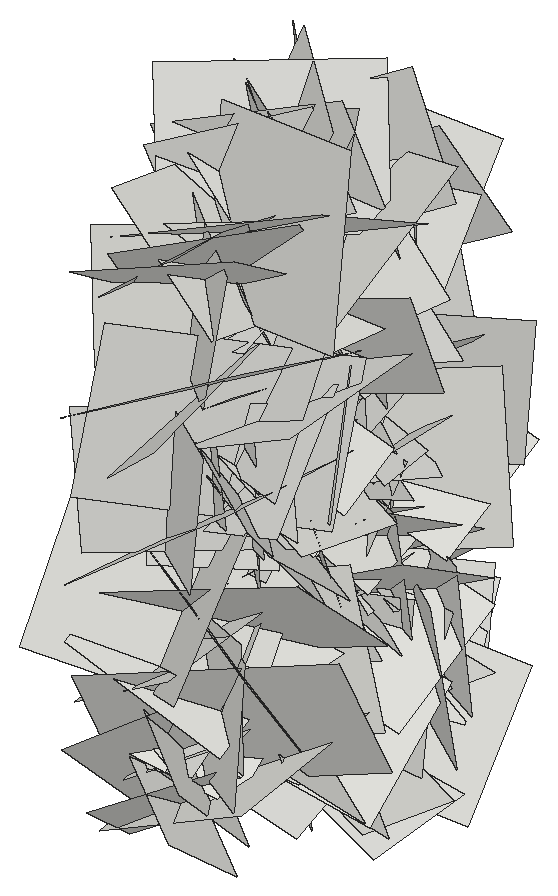
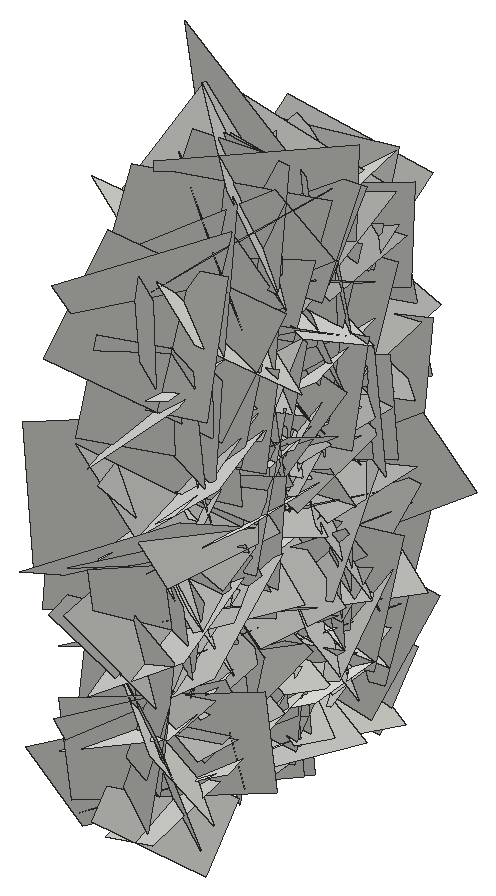
# SketchUp Ruby script. Lengths in inches.
U = 1.inch
M = Sketchup.active_model
def pt(a) = Geom::Point3d.new(a.map { |v| v * U })
def face(e, loops, mat)
  f = e.add_face(loops[0].map { |a| pt(a) })
  loops[1..].each { |l| e.add_face(l.map { |a| pt(a) }).erase! }
  f.material = f.back_material = mat if mat
  f
end
# faces: each face lists its corners as indices into pts; further lists are holes
def faces(e, pts, list, mat = nil) = list.each { |f| face(e, (f[0].is_a?(Array) ? f : [f]).map { |l| l.map { |i| pts[i] } }, mat) }
# xy, xz, yz: faces in a plane at the given z, y or x. An outline is a flat list of corners, or four numbers for a rectangle; further outlines are holes
def ring(l) = l.size == 4 ? [[l[0], l[1]], [l[2], l[1]], [l[2], l[3]], [l[0], l[3]]] : l.each_slice(2).to_a
def flat(e, list, mat, &to3) = list.each { |f| face(e, (f[0].is_a?(Array) ? f : [f]).map { |l| ring(l).map { |u, v| to3.(u, v) } }, mat) }
def xy(e, z, list, mat = nil) = flat(e, list, mat) { |x, y| [x, y, z] }
def xz(e, y, list, mat = nil) = flat(e, list, mat) { |x, z| [x, y, z] }
def yz(e, x, list, mat = nil) = flat(e, list, mat) { |y, z| [x, y, z] }
def lines(e, pts, list) = list.each { |a, b| e.add_line(pt(pts[a]), pt(pts[b])) }
# prism: a flat outline (further loops are holes) pulled along v
def prism(e, loops, v, mat = nil)
  f = face(e, loops, mat); d = Geom::Vector3d.new(v.map { |x| x * U })
  f.pushpull(f.normal.samedirection?(d) ? d.length : -d.length)
end
def box(e, o, s, mat = nil) = prism(e, [[o, [o[0] + s[0], o[1], o[2]], [o[0] + s[0], o[1] + s[1], o[2]], [o[0], o[1] + s[1], o[2]]]], [0, 0, s[2]], mat)
def at(x, y, z, deg = 0) = Geom::Transformation.translation(pt([x, y, z])) * Geom::Transformation.rotation(ORIGIN, Z_AXIS, deg.degrees)
def axes(o, x, y, z) = Geom::Transformation.new([*x, 0, *y, 0, *z, 0, *pt(o).to_a, 1])
def part(name) = M.definitions.add(name)
# library, detail: a bought-in or finely detailed component or shape, given as its bounding box
def library(name, o, s) = part(name).tap { |d| box(d.entities, o, s) }
def detail(e, o, s) = box(e.add_group.entities, o, s)
def put(e, d, t, mat = nil) = e.add_instance(d, t).tap { |i| i.material = mat if mat }
def group(e, t, mat = nil) = e.add_group.tap { |g| g.transformation = t; g.material = mat if mat }.entities
root = M.entities
c1 = part("Component\#6")
p = [[0.01,0,0],[0,3.24,4.54],[4.32,3.24,4.54],[4.33,0,0]]
faces(c1.entities,p,[[0,1,2,3]])
put(root,c1,axes([34.14,139.99,14.29],[0.01199,-0.16574,0.68191],[-0.09091,0.67656,0.16586],[0.73829,0.086,0.00935]))
put(root,c1,axes([38.11,139.9,15.42],[-0.08068,-0.00169,-0.87701],[-0.08263,-0.87681,0.00845],[-0.92595,0.07839,0.07566]))
put(root,c1,axes([34.14,145.32,5.58],[0.01721,-0.24816,-0.73855],[-0.187,-0.7207,0.23828],[0.80443,-0.16223,0.07119]))
put(root,c1,axes([38.11,140.66,10.67],[0.05387,-0.70807,-1.02445],[0.25854,-0.99979,0.70312],[-1.29449,-0.22915,0.09779]))
put(root,c1,axes([38.11,141.11,17.69],[-0.01651,0.23078,-0.87547],[-0.12637,-0.8685,-0.22682],[-0.95135,0.11136,0.04532]))
put(root,c1,axes([34.14,138.56,10.4375],[-0.05239,0.37979,0.51244],[0.10197,0.51253,-0.37059],[0.66837,-0.04842,0.0967]))
put(root,c1,axes([38.11,149.05,6.52],[0.16475,-0.3536,-1.09271],[0.00842,-1.10231,0.35784],[-1.21738,-0.05548,-0.1454]))
put(root,c1,axes([38.11,142.09,4.39],[-0.13266,-0.06807,0.83796],[-0.05074,0.84639,0.06161],[-0.88972,-0.03812,-0.12846]))
put(root,c1,axes([38.11,136.25,6.15],[-0.02753,0.62765,0.83331],[0.11118,0.83092,-0.62258],[-1.10023,0.06826,-0.08377]))
put(root,c1,axes([34.14,141.82,12.65],[0.04235,0.31596,0.66399],[-0.14644,0.65635,-0.30401],[0.76557,0.10807,-0.09488]))
put(root,c1,axes([38.11,145.41,21.68],[-0.17174,-0.50133,-0.77339],[0.12403,-0.79008,0.48764],[-0.96905,-0.01227,0.19948]))
put(root,c1,axes([34.14,139.97,19.34],[-0.20036,-0.21311,0.82685],[-0.01235,0.84743,0.21575],[0.90502,-0.03562,0.186]))
put(root,c1,axes([38.11,135.11,11.54],[0.10699,0.00448,1.06975],[-0.01257,1.07444,-0.00338],[-1.13388,-0.01149,0.10098]))
put(root,c1,axes([34.14,141.75,2.2],[0.07408,-0.19814,0.56205],[0.01701,0.56632,0.19765],[0.63148,0.00798,-0.07126]))
put(root,c1,axes([38.11,137.79,2.1],[0.03475,-0.78477,0.75119],[0.11687,0.75006,0.77877],[-1.14558,0.05272,0.10224]))
put(root,c1,axes([34.14,139.2,5.38],[-0.02645,-0.5119,-0.36479],[0.13209,-0.36186,0.49927],[0.65307,0.05245,-0.11575]))
put(root,c1,axes([38.11,139.48,6.78],[-0.1397,0.74364,0.31774],[-0.04551,0.31504,-0.75514],[-0.85599,-0.13812,-0.01171]))
put(root,c1,axes([38.11,146.4375,4.35],[0.18242,-1.06895,0.55133],[0.10581,0.56772,1.06956],[-1.27052,-0.1062,0.16823]))
put(root,c1,axes([34.14,141.96,13.08],[0.07799,-0.57044,-0.33182],[-0.05167,-0.33766,0.56968],[0.69762,0.03877,0.07929]))
put(root,c1,axes([38.11,137.55,18.4],[0.05522,0.7917,0.38208],[-0.20111,0.38385,-0.76951],[-0.90986,-0.0368,0.19328]))
put(root,c1,axes([34.14,140.67,1.375],[0.09858,-0.02009,0.69473],[-0.09996,0.69407,0.03269],[0.72991,0.09776,-0.08935]))
put(root,c1,axes([34.14,143.63,3.63],[0.04495,-0.13338,0.65571],[0.00407,0.65706,0.13341],[0.70927,0.00468,-0.04233]))
put(root,c1,axes([34.14,139.35,17.19],[0.06054,-0.33637,0.61942],[-0.0607,0.61718,0.34043],[0.74468,0.07766,-0.02261]))
put(root,c1,axes([38.11,145.52,15.88],[0.20612,-0.51117,0.96001],[-0.04532,0.97089,0.52562],[-1.15198,-0.12966,0.1511]))
put(root,c1,axes([34.14,136.74,12.93],[0.11437,0.04247,0.59628],[0.02624,0.60507,-0.04758],[0.63311,-0.03275,-0.10574]))
put(root,c1,axes([34.14,142.73,15.75],[-0.26089,1.021,-0.12695],[-0.10549,-0.15355,-1.04195],[1.08548,0.23047,-0.13178]))
put(root,c1,axes([38.11,139.41,15.5],[-0.07329,-0.02436,0.98546],[0.16551,0.97513,0.03506],[-1.03171,0.15816,-0.06438]))
put(root,c1,axes([34.14,143.53,7.33],[-0.11895,-0.88372,0.009],[-0.0734,0.01784,0.88799],[0.93392,-0.11115,0.07094]))
put(root,c1,axes([38.11,142.07,24.73],[0.13514,0.30002,-0.93652],[-0.09595,-0.93677,-0.31242],[-1.03799,0.12565,-0.09305]))
put(root,c1,axes([34.14,138.58,20.36],[-0.30182,0.3301,1.08442],[-0.18064,1.09293,-0.37743],[1.1879,0.25007,0.21813]))
put(root,c1,axes([38.11,143.76,15.19],[-0.09057,0.86782,-0.29614],[0.1091,-0.28647,-0.86917],[-0.96584,-0.11373,-0.07041]))
put(root,c1,axes([38.11,139.77,3.95],[-0.11908,-0.78329,-0.0515],[-0.03618,-0.0471,0.79084],[-0.83129,0.11425,-0.02704]))
put(root,c1,axes([34.14,146.8125,4.55],[-0.17148,-0.83232,0.10491],[0.08015,0.09194,0.84603],[0.88562,-0.16948,-0.05625]))
put(root,c1,axes([38.11,145.52,18.22],[0.02537,0.1253,-0.85934],[-0.08829,-0.85537,-0.12704],[-0.91628,0.08589,-0.01155]))
put(root,c1,axes([38.11,143.66,16.18],[-0.1105,0.58717,-0.52568],[-0.01323,-0.53143,-0.59111],[-0.83529,-0.06926,0.0789]))
put(root,c1,axes([38.11,147.01,9.44],[0.18802,-1.10018,-0.17062],[0.06994,-0.16208,1.11371],[-1.17806,-0.18521,0.03889]))
put(root,c1,axes([34.14,143.33,2.25],[0.06381,-0.71847,0.0034],[-0.02834,0.00117,0.7205],[0.76106,0.06028,0.02655]))
put(root,c1,axes([38.11,144.05,16.5],[-0.02895,-0.76847,-0.41691],[0.01722,-0.41749,0.76847],[-0.92657,0.01625,0.02731]))
put(root,c1,axes([38.11,143.95,11.7],[0.02215,-0.88691,-0.38082],[0.08723,-0.37788,0.88459],[-1.0194,-0.05161,0.06742]))
put(root,c1,axes([34.14,147.56,10.64],[0.00206,-0.13591,-0.77504],[-0.03252,-0.77447,0.13573],[0.83344,-0.02988,0.00721]))
put(root,c1,axes([34.14,142.57,12.97],[-0.12959,-0.66136,0.5647],[0.03976,0.56572,0.67067],[0.92097,-0.11748,0.0505]))
put(root,c1,axes([38.11,141.85,18.04],[0.12661,-0.3078,1.12748],[0.24587,1.11705,0.28038],[-1.21422,0.1941,0.17434]))
put(root,c1,axes([34.14,147.06,19.23],[-0.16196,0.05609,-0.92604],[0.00217,-0.93849,-0.05718],[0.9834,0.01131,-0.15239]))
put(root,c1,axes([34.14,141.5625,11.54],[-0.13399,-0.80117,0.38482],[0.02481,0.38556,0.81039],[0.9418,-0.12414,0.0334]))
put(root,c1,axes([34.14,149.3125,5.88],[-0.15882,-0.57412,-0.80425],[-0.08368,-0.80389,0.58857],[1.04409,-0.15176,-0.07517]))
put(root,c1,axes([38.11,143.03,2.65],[0.18528,-0.93043,-0.12384],[-0.14778,-0.15031,0.9325],[-0.98392,-0.15263,-0.16338]))
put(root,c1,axes([34.14,141.35,5.69],[0.05421,0.52298,-0.48745],[0.04158,-0.49001,-0.52162],[0.75668,-0.01054,0.06359]))
put(root,c1,axes([38.11,145.65,3.28],[-0.1646,0.60158,-0.34623],[-0.0091,-0.35642,-0.61544],[-0.73568,-0.13018,0.08507]))
put(root,c1,axes([34.14,139.62,7.21],[-0.15609,-0.9187,-0.23757],[-0.00588,-0.23958,0.92989],[1.00583,-0.14396,-0.03143]))
put(root,c1,axes([34.14,143.17,8.1],[0.04482,0.75985,0.07181],[0.00358,0.07173,-0.76102],[0.80902,-0.04241,-0.00061]))
put(root,c1,axes([34.14,141.47,13.3125],[-0.15098,-0.93805,0.13539],[-0.00567,0.13771,0.94846],[1.00463,-0.1402,0.0257]))
put(root,c1,axes([38.11,139.94,18.75],[0.02341,-0.9115,0.17831],[0.09444,0.17962,0.90714],[-0.97996,-0.00447,0.09169]))
put(root,c1,axes([34.14,144.39,10.35],[-0.12238,0.87118,-0.30871],[-0.00416,-0.31157,-0.87778],[0.97971,0.1075,-0.04229]))
put(root,c1,axes([34.14,135.6875,17.375],[-0.11773,0.10526,0.9962],[-0.108,0.99592,-0.11659],[1.05635,0.11356,0.09911]))
put(root,c1,axes([34.14,136.7,5.12],[0.11008,0.58852,-0.4619],[-0.03608,-0.46213,-0.59646],[0.7922,-0.10282,0.03702]))
put(root,c1,axes([38.11,147.32,10.4375],[0.06119,-0.47987,-0.75245],[0.01649,-0.75336,0.48165],[-0.94584,-0.04418,-0.04028]))
put(root,c1,axes([34.14,147.32,10.4375],[-0.06119,-0.47987,-0.75245],[-0.01649,-0.75336,0.48165],[0.94584,-0.04418,-0.04028]))
put(root,c1,axes([38.11,136.7,5.12],[-0.11008,0.58852,-0.4619],[0.03608,-0.46213,-0.59646],[-0.7922,-0.10282,0.03702]))
put(root,c1,axes([38.11,135.6875,17.375],[0.11773,0.10526,0.9962],[0.108,0.99592,-0.11659],[-1.05635,0.11356,0.09911]))
put(root,c1,axes([38.11,144.39,10.35],[0.12238,0.87118,-0.30871],[0.00416,-0.31157,-0.87778],[-0.97971,0.1075,-0.04229]))
put(root,c1,axes([34.14,139.94,18.75],[-0.02341,-0.9115,0.17831],[-0.09444,0.17962,0.90714],[0.97996,-0.00447,0.09169]))
put(root,c1,axes([38.11,141.47,13.3125],[0.15098,-0.93805,0.13539],[0.00567,0.13771,0.94846],[-1.00463,-0.1402,0.0257]))
put(root,c1,axes([38.11,143.17,8.1],[-0.04482,0.75985,0.07181],[-0.00358,0.07173,-0.76102],[-0.80902,-0.04241,-0.00061]))
put(root,c1,axes([38.11,139.62,7.21],[0.15609,-0.9187,-0.23757],[0.00588,-0.23958,0.92989],[-1.00583,-0.14396,-0.03143]))
put(root,c1,axes([34.14,145.65,3.28],[0.1646,0.60158,-0.34623],[0.0091,-0.35642,-0.61544],[0.73568,-0.13018,0.08507]))
put(root,c1,axes([38.11,141.35,5.69],[-0.05421,0.52298,-0.48745],[-0.04158,-0.49001,-0.52162],[-0.75668,-0.01054,0.06359]))
put(root,c1,axes([34.14,143.03,2.65],[-0.18528,-0.93043,-0.12384],[0.14778,-0.15031,0.9325],[0.98392,-0.15263,-0.16338]))
put(root,c1,axes([38.11,149.3125,5.88],[0.15882,-0.57412,-0.80425],[0.08368,-0.80389,0.58857],[-1.04409,-0.15176,-0.07517]))
put(root,c1,axes([38.11,141.5625,11.54],[0.13399,-0.80117,0.38482],[-0.02481,0.38556,0.81039],[-0.9418,-0.12414,0.0334]))
put(root,c1,axes([38.11,147.06,19.23],[0.16196,0.05609,-0.92604],[-0.00217,-0.93849,-0.05718],[-0.9834,0.01131,-0.15239]))
put(root,c1,axes([34.14,141.85,18.04],[-0.12661,-0.3078,1.12748],[-0.24587,1.11705,0.28038],[1.21422,0.1941,0.17434]))
put(root,c1,axes([38.11,142.57,12.97],[0.12959,-0.66136,0.5647],[-0.03976,0.56572,0.67067],[-0.92097,-0.11748,0.0505]))
put(root,c1,axes([38.11,147.56,10.64],[-0.00206,-0.13591,-0.77504],[0.03252,-0.77447,0.13573],[-0.83344,-0.02988,0.00721]))
put(root,c1,axes([34.14,143.95,11.7],[-0.02215,-0.88691,-0.38082],[-0.08723,-0.37788,0.88459],[1.0194,-0.05161,0.06742]))
put(root,c1,axes([34.14,144.05,16.5],[0.02895,-0.76847,-0.41691],[-0.01722,-0.41749,0.76847],[0.92657,0.01625,0.02731]))
put(root,c1,axes([38.11,143.33,2.25],[-0.06381,-0.71847,0.0034],[0.02834,0.00117,0.7205],[-0.76106,0.06028,0.02655]))
put(root,c1,axes([34.14,147.01,9.44],[-0.18802,-1.10018,-0.17062],[-0.06994,-0.16208,1.11371],[1.17806,-0.18521,0.03889]))
put(root,c1,axes([34.14,143.66,16.18],[0.1105,0.58717,-0.52568],[0.01323,-0.53143,-0.59111],[0.83529,-0.06926,0.0789]))
put(root,c1,axes([34.14,145.52,18.22],[-0.02537,0.1253,-0.85934],[0.08829,-0.85537,-0.12704],[0.91628,0.08589,-0.01155]))
put(root,c1,axes([38.11,133.42,16.97],[0.14677,0.94615,0.46149],[0.22557,0.4307,-0.94687],[-1.09283,0.21597,-0.13346]))
put(root,c1,axes([38.11,146.8125,4.55],[0.17148,-0.83232,0.10491],[-0.08015,0.09194,0.84603],[-0.88562,-0.16948,-0.05625]))
put(root,c1,axes([34.14,139.77,3.95],[0.11908,-0.78329,-0.0515],[0.03618,-0.0471,0.79084],[0.83129,0.11425,-0.02704]))
put(root,c1,axes([34.14,143.76,15.19],[0.09057,0.86782,-0.29614],[-0.1091,-0.28647,-0.86917],[0.96584,-0.11373,-0.07041]))
put(root,c1,axes([38.11,138.58,20.36],[0.30182,0.3301,1.08442],[0.18064,1.09293,-0.37743],[-1.1879,0.25007,0.21813]))
put(root,c1,axes([34.14,142.07,24.73],[-0.13514,0.30002,-0.93652],[0.09595,-0.93677,-0.31242],[1.03799,0.12565,-0.09305]))
put(root,c1,axes([38.11,143.53,7.33],[0.11895,-0.88372,0.009],[0.0734,0.01784,0.88799],[-0.93392,-0.11115,0.07094]))
put(root,c1,axes([34.14,139.41,15.5],[0.07329,-0.02436,0.98546],[-0.16551,0.97513,0.03506],[1.03171,0.15816,-0.06438]))
put(root,c1,axes([38.11,142.73,15.75],[0.26089,1.021,-0.12695],[0.10549,-0.15355,-1.04195],[-1.08548,0.23047,-0.13178]))
put(root,c1,axes([38.11,136.74,12.93],[-0.11437,0.04247,0.59628],[-0.02624,0.60507,-0.04758],[-0.63311,-0.03275,-0.10574]))
put(root,c1,axes([34.14,145.52,15.88],[-0.20612,-0.51117,0.96001],[0.04532,0.97089,0.52562],[1.15198,-0.12966,0.1511]))
put(root,c1,axes([38.11,139.35,17.19],[-0.06054,-0.33637,0.61942],[0.0607,0.61718,0.34043],[-0.74468,0.07766,-0.02261]))
put(root,c1,axes([38.11,143.63,3.63],[-0.04495,-0.13338,0.65571],[-0.00407,0.65706,0.13341],[-0.70927,0.00468,-0.04233]))
put(root,c1,axes([38.11,140.67,1.375],[-0.09858,-0.02009,0.69473],[0.09996,0.69407,0.03269],[-0.72991,0.09776,-0.08935]))
put(root,c1,axes([34.14,137.55,18.4],[-0.05522,0.7917,0.38208],[0.20111,0.38385,-0.76951],[0.90986,-0.0368,0.19328]))
put(root,c1,axes([38.11,141.96,13.08],[-0.07799,-0.57044,-0.33182],[0.05167,-0.33766,0.56968],[-0.69762,0.03877,0.07929]))
put(root,c1,axes([34.14,146.4375,4.35],[-0.18242,-1.06895,0.55133],[-0.10581,0.56772,1.06956],[1.27052,-0.1062,0.16823]))
put(root,c1,axes([34.14,139.48,6.78],[0.1397,0.74364,0.31774],[0.04551,0.31504,-0.75514],[0.85599,-0.13812,-0.01171]))
put(root,c1,axes([38.11,139.2,5.38],[0.02645,-0.5119,-0.36479],[-0.13209,-0.36186,0.49927],[-0.65307,0.05245,-0.11575]))
put(root,c1,axes([34.14,137.79,2.1],[-0.03475,-0.78477,0.75119],[-0.11687,0.75006,0.77877],[1.14558,0.05272,0.10224]))
put(root,c1,axes([38.11,141.75,2.2],[-0.07408,-0.19814,0.56205],[-0.01701,0.56632,0.19765],[-0.63148,0.00798,-0.07126]))
put(root,c1,axes([34.14,135.11,11.54],[-0.10699,0.00448,1.06975],[0.01257,1.07444,-0.00338],[1.13388,-0.01149,0.10098]))
put(root,c1,axes([38.11,139.97,19.34],[0.20036,-0.21311,0.82685],[0.01235,0.84743,0.21575],[-0.90502,-0.03562,0.186]))
put(root,c1,axes([34.14,145.41,21.68],[0.17174,-0.50133,-0.77339],[-0.12403,-0.79008,0.48764],[0.96905,-0.01227,0.19948]))
put(root,c1,axes([38.11,141.82,12.65],[-0.04235,0.31596,0.66399],[0.14644,0.65635,-0.30401],[-0.76557,0.10807,-0.09488]))
put(root,c1,axes([34.14,136.25,6.15],[0.02753,0.62765,0.83331],[-0.11118,0.83092,-0.62258],[1.10023,0.06826,-0.08377]))
put(root,c1,axes([34.14,142.09,4.39],[0.13266,-0.06807,0.83796],[0.05074,0.84639,0.06161],[0.88972,-0.03812,-0.12846]))
put(root,c1,axes([34.14,149.05,6.52],[-0.16475,-0.3536,-1.09271],[-0.00842,-1.10231,0.35784],[1.21738,-0.05548,-0.1454]))
put(root,c1,axes([38.11,138.56,10.4375],[0.05239,0.37979,0.51244],[-0.10197,0.51253,-0.37059],[-0.66837,-0.04842,0.0967]))
put(root,c1,axes([34.14,141.11,17.69],[0.01651,0.23078,-0.87547],[0.12637,-0.8685,-0.22682],[0.95135,0.11136,0.04532]))
put(root,c1,axes([34.14,140.66,10.67],[-0.05387,-0.70807,-1.02445],[-0.25854,-0.99979,0.70312],[1.29449,-0.22915,0.09779]))
put(root,c1,axes([38.11,145.32,5.58],[-0.01721,-0.24816,-0.73855],[0.187,-0.7207,0.23828],[-0.80443,-0.16223,0.07119]))
put(root,c1,axes([34.14,139.9,15.42],[0.08068,-0.00169,-0.87701],[0.08263,-0.87681,0.00845],[0.92595,0.07839,0.07566]))
put(root,c1,axes([38.11,139.99,14.29],[-0.01199,-0.16574,0.68191],[0.09091,0.67656,0.16586],[-0.73829,0.086,0.00935]))
put(root,c1,axes([38.11,147.58,14.43],[0.15626,-0.88067,0.15465],[0.14549,0.17716,0.87807],[-0.93656,-0.11942,0.1622]))
put(root,c1,axes([38.11,138.3,10.21],[0.07821,-0.14386,0.79141],[0.12147,0.78851,0.13265],[-0.84394,0.10016,0.09244]))
put(root,c1,axes([34.14,142.2,15.72],[-0.2001,0.61396,-1.10583],[-0.10306,-1.12181,-0.60624],[1.33676,0.00542,-0.21228]))
put(root,c1,axes([34.14,141.25,1.55],[0.11713,-0.0063,1.0149],[-0.13715,1.01248,0.02037],[1.06704,0.13083,-0.10878]))
put(root,c1,axes([34.14,144.34,6.82],[-0.01542,0.93301,-0.17325],[0.14993,-0.1692,-0.92309],[0.99466,0.03997,0.13646]))
put(root,c1,axes([34.14,137.99,14.66],[-0.08461,-0.27233,0.9902],[0.1352,0.98287,0.28059],[1.08015,-0.14435,0.04245]))
put(root,c1,axes([34.14,142.29,19.52],[0.02505,0.60517,0.90894],[-0.1077,0.90642,-0.60085],[1.15246,0.07156,-0.07591]))
put(root,c1,axes([34.14,144.58,9.97],[0.16827,0.58944,-0.69808],[-0.0398,-0.70373,-0.60275],[0.96765,-0.13145,0.0966]))
put(root,c1,axes([38.11,139.8125,20.98],[-0.02151,0.52563,-0.34386],[0.05265,-0.34162,-0.52514],[-0.66372,-0.04413,-0.03051]))
put(root,c1,axes([38.11,142.6,14.22],[0.18899,-0.6396,-0.42028],[-0.00285,-0.43205,0.65638],[-0.81124,-0.14749,-0.10022]))
put(root,c1,axes([38.11,145.36,10.15],[0.14636,-0.64891,0.3527],[0.01811,0.36152,0.65845],[-0.78267,-0.11298,0.08119]))
put(root,c1,axes([38.11,145.42,18.19],[0.07853,-0.05807,0.70782],[0.06912,0.70921,0.05136],[-0.74963,0.05931,0.07889]))
put(root,c1,axes([34.14,146.45,10.34],[0.10559,0.05407,-0.92917],[0.0532,-0.93343,-0.04894],[0.98516,0.04461,0.10223]))
put(root,c1,axes([38.11,141.95,12.73],[0.09992,0.55515,0.3498],[-0.02862,0.35638,-0.5583],[-0.69495,0.06514,0.07329]))
put(root,c1,axes([34.14,137.63,3.85],[-0.23328,-0.07655,1.22947],[0.08564,1.24535,0.092],[1.30295,-0.09556,0.21407]))
put(root,c1,axes([34.14,137.89,18.97],[0.02244,-0.79516,0.48934],[0.22215,0.48102,0.77258],[0.96443,-0.0923,-0.18934]))
put(root,c1,axes([38.11,139.18,13.74],[0.11062,-0.13563,-0.63299],[-0.03095,-0.6415,0.13263],[-0.6855,0.00708,-0.10814]))
put(root,c1,axes([34.14,141.92,3.18],[0.02887,1.0089,0.10446],[0.06921,0.10254,-1.00735],[1.07292,-0.03376,0.06217]))
put(root,c1,axes([34.14,138.34,13.4],[0.1901,0.66514,0.65147],[-0.02496,0.66648,-0.67398],[0.98658,-0.1113,-0.14258]))
put(root,c1,axes([34.14,138.76,9.15],[0.08107,-0.07376,-0.93469],[0.12107,-0.93007,0.08274],[0.98644,0.12021,0.06666]))
put(root,c1,axes([34.14,139.52,8.83],[0.01584,-0.12995,-1.07448],[0.00128,-1.07458,0.12998],[1.14724,0.003,0.01469]))
put(root,c1,axes([34.14,137.41,10.49],[0.17918,0.96529,0.20208],[-0.06958,0.21558,-0.97489],[1.04307,-0.15144,-0.09975]))
put(root,c1,axes([34.14,141.07,4.77],[-0.0925,1.07709,-0.24358],[0.13853,-0.23255,-1.07513],[1.16232,0.11343,0.10875]))
put(root,c1,axes([34.14,143.54,11.83],[-0.01207,0.98557,0.48784],[0.03058,0.48797,-0.98515],[1.16528,-0.0026,0.03091]))
put(root,c1,axes([38.11,142.82,6.12],[-0.04161,-0.60559,-0.03198],[0.13563,-0.03959,0.59276],[-0.62835,0.03156,0.13006]))
put(root,c1,axes([34.14,142.72,8.07],[-0.13823,0.05764,1.30603],[-0.0986,1.30878,-0.06705],[1.38223,0.09912,0.12583]))
put(root,c1,axes([34.14,138.64,15.1],[-0.05154,1.07135,-0.23626],[0.10153,-0.23144,-1.06922],[1.15847,0.06794,0.08319]))
put(root,c1,axes([34.14,138.49,4.97],[-0.13436,1.04009,0.6085],[0.04809,0.61554,-1.04268],[1.27641,0.08629,0.10334]))
put(root,c1,axes([38.11,137.29,3.46],[0.14224,0.61257,0.15159],[-0.04066,0.16261,-0.62315],[-0.66768,0.1206,0.07024]))
put(root,c1,axes([34.14,137.21,11.6875],[-0.11385,0.72886,-0.88593],[0.14818,-0.87485,-0.7367],[1.20699,0.17615,0.00688]))
put(root,c1,axes([34.14,143.17,19.13],[0.20193,0.9279,-0.28366],[0.04691,-0.29708,-0.94209],[1.02744,-0.16881,0.09877]))
put(root,c1,axes([34.14,142.88,1.98],[0.0351,0.64216,0.95117],[0.00533,0.95147,-0.64254],[1.21649,-0.02269,-0.02463]))
put(root,c1,axes([34.14,137.64,18.89],[0.26376,-0.64139,0.69016],[0.02251,0.71746,0.65911],[0.99845,0.15326,-0.19718]))
put(root,c1,axes([34.14,140.93,18.6875],[-0.10901,-0.41314,-1.06231],[0.28274,-1.04573,0.38087],[1.17466,0.21337,-0.19026]))
put(root,c1,axes([34.14,141.75,2.91],[-0.11729,-1.19784,-0.30033],[0.11289,-0.30967,1.19584],[1.30414,-0.08092,-0.13053]))
put(root,c1,axes([34.14,143.08,17.68],[-0.06532,-0.13436,-1.17102],[0.13166,-1.16683,0.12734],[1.24247,0.11658,-0.07506]))
put(root,c1,axes([34.14,140.04,10.48],[-0.03722,-1.27767,0.05021],[-0.04996,0.05148,1.27723],[1.35446,-0.03321,0.04849]))
put(root,c1,axes([34.14,140.59,7.56],[-0.03383,1.06332,0.50099],[0.10932,0.50178,-1.05842],[1.24115,-0.01522,0.10688]))
put(root,c1,axes([34.14,137.94,15.45],[-0.03401,0.89045,-0.73196],[0.17038,-0.72163,-0.88493],[1.2099,0.12665,0.10405]))
put(root,c1,axes([34.14,146.96,20.2],[-0.19126,-1.0536,-0.82739],[0.10265,-0.84293,1.05228],[1.41631,-0.08119,-0.188]))
put(root,c1,axes([34.14,139.77,22.87],[0.12093,1.26112,-0.05281],[-0.18505,-0.03675,-1.25475],[1.32509,-0.12022,-0.17041]))
put(root,c1,axes([34.14,139.44,14.86],[-0.04621,-1.16691,0.31838],[0.12643,0.31289,1.16311],[1.27589,-0.07327,-0.10372]))
put(root,c1,axes([34.14,141.48,7.17],[0.20337,0.82379,-0.77749],[-0.08888,-0.77608,-0.84298],[1.19742,-0.19752,0.06948]))
put(root,c1,axes([34.14,138.37,16.22],[0.07456,0.76169,-0.90937],[0.0504,-0.91204,-0.76025],[1.25638,-0.00862,0.08446]))
put(root,c1,axes([34.14,148.05,8.79],[0.07068,0.0827,-1.14811],[0.1221,-1.14474,-0.07576],[1.21402,0.11031,0.07447]))
put(root,c1,axes([34.14,144.3,10.94],[0.16969,-0.07735,1.18237],[-0.06112,1.19119,0.08573],[1.2545,0.0685,-0.15576]))
put(root,c1,axes([34.14,144.73,5.33],[0.04426,-1.02294,0.56209],[0.16257,0.56238,1.01208],[1.2265,-0.03763,-0.15444]))
put(root,c1,axes([34.14,141.11,14.91],[0.10517,-0.78429,-0.79452],[0.18451,-0.77703,0.78876],[1.16892,0.19321,-0.05302]))
put(root,c1,axes([34.14,134.59,13.6],[0.14779,0.17555,1.29716],[-0.16453,1.29751,-0.15892],[1.37773,0.13612,-0.15813]))
put(root,c1,axes([34.14,148.13,7.79],[0.13698,0.11741,-1.23467],[-0.05668,-1.23967,-0.12348],[1.31343,-0.06574,0.12344]))
put(root,c1,axes([34.14,139.3125,6.46],[-0.05297,-0.89114,0.82127],[0.332,0.78454,0.87035],[1.24093,-0.24794,-0.1978]))
put(root,c1,axes([34.14,142.16,14.375],[-0.02255,-1.26636,-0.09652],[0.2141,-0.09868,1.25016],[1.3291,-0.00559,-0.20302]))
put(root,c1,axes([34.14,141.32,18.93],[-0.00931,-1.12138,0.55372],[0.26786,0.54072,1.09906],[1.29833,-0.1196,-0.22278]))
put(root,c1,axes([34.14,140.96,14.21],[0.1647,-0.56811,1.02456],[0.16232,1.03452,0.5504],[1.23116,-0.0604,-0.20963]))
put(root,c1,axes([34.14,137.06,3.09],[0.11239,-0.69918,1.17187],[0.18512,1.17269,0.68387],[1.43458,-0.09655,-0.18006]))
put(root,c1,axes([34.14,141.18,23.91],[0.20239,-0.45291,-1.29893],[0.24414,-1.28235,0.48098],[1.43758,0.28153,0.10118]))
